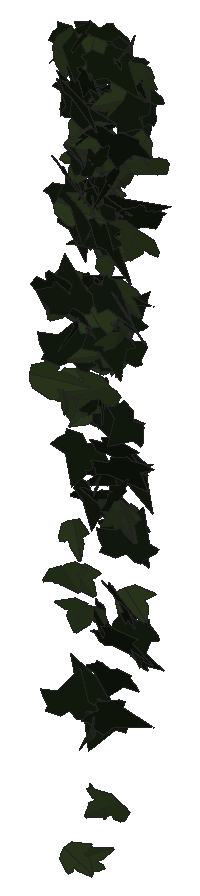
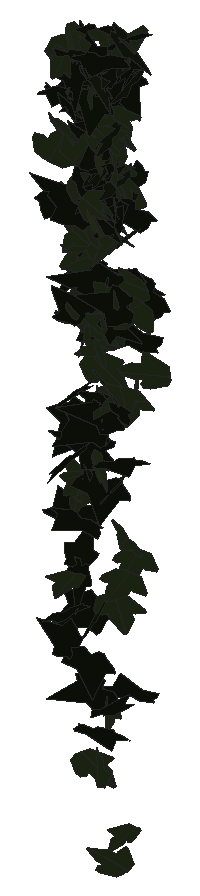
# SketchUp Ruby script. Lengths in inches.
U = 1.inch
M = Sketchup.active_model
def pt(a) = Geom::Point3d.new(a.map { |v| v * U })
def face(e, loops, mat)
  f = e.add_face(loops[0].map { |a| pt(a) })
  loops[1..].each { |l| e.add_face(l.map { |a| pt(a) }).erase! }
  f.material = f.back_material = mat if mat
  f
end
# faces: each face lists its corners as indices into pts; further lists are holes
def faces(e, pts, list, mat = nil) = list.each { |f| face(e, (f[0].is_a?(Array) ? f : [f]).map { |l| l.map { |i| pts[i] } }, mat) }
# xy, xz, yz: faces in a plane at the given z, y or x. An outline is a flat list of corners, or four numbers for a rectangle; further outlines are holes
def ring(l) = l.size == 4 ? [[l[0], l[1]], [l[2], l[1]], [l[2], l[3]], [l[0], l[3]]] : l.each_slice(2).to_a
def flat(e, list, mat, &to3) = list.each { |f| face(e, (f[0].is_a?(Array) ? f : [f]).map { |l| ring(l).map { |u, v| to3.(u, v) } }, mat) }
def xy(e, z, list, mat = nil) = flat(e, list, mat) { |x, y| [x, y, z] }
def xz(e, y, list, mat = nil) = flat(e, list, mat) { |x, z| [x, y, z] }
def yz(e, x, list, mat = nil) = flat(e, list, mat) { |y, z| [x, y, z] }
def lines(e, pts, list) = list.each { |a, b| e.add_line(pt(pts[a]), pt(pts[b])) }
# prism: a flat outline (further loops are holes) pulled along v
def prism(e, loops, v, mat = nil)
  f = face(e, loops, mat); d = Geom::Vector3d.new(v.map { |x| x * U })
  f.pushpull(f.normal.samedirection?(d) ? d.length : -d.length)
end
def box(e, o, s, mat = nil) = prism(e, [[o, [o[0] + s[0], o[1], o[2]], [o[0] + s[0], o[1] + s[1], o[2]], [o[0], o[1] + s[1], o[2]]]], [0, 0, s[2]], mat)
def at(x, y, z, deg = 0) = Geom::Transformation.translation(pt([x, y, z])) * Geom::Transformation.rotation(ORIGIN, Z_AXIS, deg.degrees)
def axes(o, x, y, z) = Geom::Transformation.new([*x, 0, *y, 0, *z, 0, *pt(o).to_a, 1])
def part(name) = M.definitions.add(name)
# library, detail: a bought-in or finely detailed component or shape, given as its bounding box
def library(name, o, s) = part(name).tap { |d| box(d.entities, o, s) }
def detail(e, o, s) = box(e.add_group.entities, o, s)
def put(e, d, t, mat = nil) = e.add_instance(d, t).tap { |i| i.material = mat if mat }
def group(e, t, mat = nil) = e.add_group.tap { |g| g.transformation = t; g.material = mat if mat }.entities
root = M.entities
M.materials.add("1026 AP 7946 SUNNY SIDE UP").color = [254, 231, 186]
M.materials.add("efeu1").color = [18, 25, 13]
M.materials.add("efeu2").color = [43, 57, 29]
c1 = part("ivyleaf_9")
p = [[1.54,2.16,1.25],[1.36,2.04,1.19],[-0.21,0.99,0.68],[-0.71,1.11,0.82],[-0.85,0.86,0.67],[-0.8,0.17,0.21],
  [-0.9,-0.01,0.1],[-0.67,-0.16,-0.02],[-0.08,-0.08,-0.05],[-0.03,-0.6,-0.4],[0.65,-0.88,-0.66],[0.83,-0.6,-0.49],
  [1.29,-0.42,-0.43],[1.8125,-0.07,-0.26],[1.21,0.44,0.15]]
faces(c1.entities,p,[[0,1,2,3,4,5,6,7,8,9,10,11,12,13,14]],"efeu1")
c2 = part("ivyleaf_10")
p = [[0,0.5,-0.03],[-0.0625,2.02,-0.43],[-0.19,2.01,-0.46],[-0.54,1.05,-0.29],[-0.52,0.625,-0.18],[-0.83,0.76,-0.28],
  [-1.16,0.64,-0.33],[-1.15,0.33,-0.24],[-0.77,-0.39,0.02],[-0.3,-0.51,0.16],[0.04,-0.48,0.23],[-0.02,2.01,-0.4375],
  [-0.06,2.01,-0.43],[0.04,-0.49,0.23],[0.67,-0.49,0.14],[1.38,0.36,-0.2],[1.375,0.51,-0.24],[0.81,0.65,-0.19],
  [0.62,0.59,-0.15],[0.6,1.09,-0.28],[0.5,1.23,-0.31]]
faces(c2.entities,p,[[0,1,2,3,4,5,6,7,8,9,10],[11,12,0,13,14,15,16,17,18,19,20]],"efeu2")
put(root,c1,axes([114.33,211.82,262.76],[-0.00033,-0.02654,-0.29608],[0.42879,0.09367,-0.00857],[0.14794,-0.27155,0.02419]),"1026 AP 7946 SUNNY SIDE UP")
put(root,c2,axes([114.36,211.6,260.97],[0.01254,0.02681,0.3018],[0.335,0.20134,-0.02379],[-0.31863,0.21274,-0.01313]),"1026 AP 7946 SUNNY SIDE UP")
put(root,c1,axes([114.53,212.3125,263.96],[0.05283,-0.25311,0.0512],[0.00752,-0.05095,-0.26333],[0.40596,0.03388,-0.00179]),"1026 AP 7946 SUNNY SIDE UP")
put(root,c1,axes([114.43,212.23,264.58],[0.0163,-0.07375,-0.26726],[0.20241,0.22903,-0.06054],[0.37195,-0.1214,0.04466]),"1026 AP 7946 SUNNY SIDE UP")
put(root,c2,axes([114.68,212.33,265.17],[0.37543,-0.0503,-0.0193],[-0.0357,-0.01866,-0.25037],[0.0763,0.23875,-0.02217]),"1026 AP 7946 SUNNY SIDE UP")
put(root,c1,axes([114.86,212.49,254.3],[-0.23794,-0.17805,0.07517],[0.05656,0.06631,0.24062],[-0.29784,0.15483,-0.01435]),"1026 AP 7946 SUNNY SIDE UP")
put(root,c2,axes([114.63,211.9375,260.46],[-0.16039,0.14591,0.17325],[0.16301,-0.13156,0.1825],[0.30873,0.14527,-0.00635]),"1026 AP 7946 SUNNY SIDE UP")
put(root,c2,axes([114.74,211.63,267.7],[-0.08324,0.20278,0.25563],[-0.10928,0.23706,-0.21446],[-0.49046,-0.08723,0.0044]),"1026 AP 7946 SUNNY SIDE UP")
put(root,c2,axes([114.67,212.23,260.8],[0.36793,0.07961,-0.01973],[-0.01745,-0.02801,-0.2537],[-0.12773,0.23313,-0.02219]),"1026 AP 7946 SUNNY SIDE UP")
put(root,c1,axes([114.54,212.54,265.16],[0.08372,-0.2346,0.12588],[0.04917,-0.11956,-0.2485],[0.41398,0.06164,0.00406]),"1026 AP 7946 SUNNY SIDE UP")
put(root,c1,axes([114.47,212.09,264.97],[0.21612,-0.20264,0.12668],[0.08618,-0.11248,-0.25238],[0.36358,0.14712,-0.01548]),"1026 AP 7946 SUNNY SIDE UP")
put(root,c2,axes([114.53,212.5625,265.2],[0.08758,-0.0713,0.2423],[0.29426,-0.14466,-0.09152],[0.25145,0.19413,0.02271]),"1026 AP 7946 SUNNY SIDE UP")
put(root,c2,axes([114.8,211.98,260.54],[-0.40626,-0.08288,0.02084],[-0.01696,-0.03377,-0.27815],[0.13324,-0.25699,0.02815]),"1026 AP 7946 SUNNY SIDE UP")
put(root,c1,axes([114.6,212.53,264.3],[-0.03694,-0.00983,0.26946],[0.05812,-0.26016,-0.00817],[0.40753,0.03621,0.02559]),"1026 AP 7946 SUNNY SIDE UP")
put(root,c1,axes([114.89,212.07,267.89],[-0.28619,0.1571,-0.11604],[0.10185,-0.09749,-0.24652],[-0.28726,-0.19108,0.02821]),"1026 AP 7946 SUNNY SIDE UP")
put(root,c1,axes([114.73,212.36,259.39],[-0.23447,-0.21161,-0.00629],[0.02595,-0.00564,-0.26616],[0.33181,-0.14909,0.01637]),"1026 AP 7946 SUNNY SIDE UP")
put(root,c1,axes([114.58,212.3,262.59],[0.12474,0.16786,-0.16247],[0.02669,0.16306,0.18742],[0.3622,-0.06983,0.04214]),"1026 AP 7946 SUNNY SIDE UP")
put(root,c2,axes([114.64,212.38,264.49],[0.21264,-0.16234,0.19252],[0.18389,-0.14697,-0.2185],[0.34429,0.17876,-0.0022]),"1026 AP 7946 SUNNY SIDE UP")
put(root,c2,axes([114.59,211.98,262.4],[-0.28318,-0.13528,-0.22766],[0.31958,0.09168,-0.22871],[0.25105,-0.2693,0.03435]),"1026 AP 7946 SUNNY SIDE UP")
put(root,c2,axes([114.7,212.1,256.93],[-0.28135,-0.14537,-0.11809],[0.17248,0.04376,-0.235],[0.23349,-0.20749,0.03131]),"1026 AP 7946 SUNNY SIDE UP")
put(root,c2,axes([114.61,212.15,257.77],[0.30253,-0.05646,0.16587],[0.22686,-0.07661,-0.20532],[0.14411,0.23911,-0.025]),"1026 AP 7946 SUNNY SIDE UP")
put(root,c1,axes([114.84,211.77,254.35],[-0.32827,0.01537,0.1306],[0.20064,0.02171,0.21404],[0.00283,0.24323,-0.02592]),"1026 AP 7946 SUNNY SIDE UP")
put(root,c2,axes([114.78,211.7,257.17],[-0.25204,-0.16994,-0.10612],[0.13137,0.06108,-0.23964],[0.28264,-0.17993,0.01676]),"1026 AP 7946 SUNNY SIDE UP")
put(root,c2,axes([114.98,212.04,256.31],[-0.37933,-0.09776,0.08145],[-0.10045,-0.05342,-0.26729],[0.17091,-0.24836,0.02369]),"1026 AP 7946 SUNNY SIDE UP")
put(root,c1,axes([114.77,212.05,267.81],[-0.09165,-0.25481,0.01381],[0.00442,-0.01587,-0.2693],[0.40131,-0.05802,0.00612]),"1026 AP 7946 SUNNY SIDE UP")
put(root,c2,axes([114.8125,212.31,263.83],[-0.01325,0.17298,0.19125],[-0.0111,0.18453,-0.17733],[-0.3977,-0.01092,-0.00142]),"1026 AP 7946 SUNNY SIDE UP")
put(root,c2,axes([114.97,212.18,265.3],[-0.42627,0.09776,-0.06355],[-0.08046,0.0411,0.29635],[0.1635,0.27509,-0.01985]),"1026 AP 7946 SUNNY SIDE UP")
put(root,c1,axes([115.01,211.63,262.65],[-0.44689,0.03987,0.0216],[0.03714,0.01954,0.29485],[0.06012,0.28429,-0.02159]),"1026 AP 7946 SUNNY SIDE UP")
put(root,c2,axes([115.05,212.33,265.92],[-0.24515,-0.10156,0.16635],[-0.14571,-0.14278,-0.18486],[0.26306,-0.17373,0.05263]),"1026 AP 7946 SUNNY SIDE UP")
put(root,c2,axes([115.02,212.12,266.26],[-0.29988,-0.12456,0.12883],[-0.09785,-0.12589,-0.22639],[0.26055,-0.19063,0.06326]),"1026 AP 7946 SUNNY SIDE UP")
put(root,c1,axes([115.02,212.05,266.45],[0.10534,0.08239,0.2645],[-0.36305,-0.1182,0.10063],[0.21764,-0.23705,0.03985]),"1026 AP 7946 SUNNY SIDE UP")
put(root,c2,axes([114.58,211.92,262.8125],[-0.04554,-0.04058,-0.28364],[0.41006,-0.09998,-0.01367],[-0.15179,-0.25792,0.04816]),"1026 AP 7946 SUNNY SIDE UP")
put(root,c1,axes([114.76,212.37,265.35],[0.04224,-0.16714,-0.2027],[0.01587,0.19741,-0.17101],[0.4045,0.00971,0.02788]),"1026 AP 7946 SUNNY SIDE UP")
put(root,c2,axes([114.76,212.2,251.09],[-0.15756,-0.10948,0.19911],[0.17686,0.15862,0.15308],[-0.30217,0.14992,-0.01423]),"1026 AP 7946 SUNNY SIDE UP")
put(root,c1,axes([115,212.14,262.17],[-0.13648,0.11021,-0.22666],[0.13675,-0.2052,-0.14204],[-0.3629,-0.11877,0.03171]),"1026 AP 7946 SUNNY SIDE UP")
put(root,c1,axes([114.91,211.74,261.48],[-0.38073,0.00603,0.1913],[0.29141,-0.0128,0.24935],[0.01977,0.30485,0.00848]),"1026 AP 7946 SUNNY SIDE UP")
put(root,c2,axes([115.02,212.24,260.35],[0.16107,0.12713,-0.20432],[-0.17254,-0.16652,-0.16871],[-0.32888,0.14963,-0.01156]),"1026 AP 7946 SUNNY SIDE UP")
put(root,c2,axes([114.92,212.52,265.6],[0.06572,-0.21079,0.17182],[0.08258,-0.16036,-0.2217],[0.4157,0.06518,0.01688]),"1026 AP 7946 SUNNY SIDE UP")
put(root,c1,axes([114.97,212.62,253.97],[-0.31181,-0.13764,-0.05804],[0.08965,0.01497,-0.24776],[0.21548,-0.2054,0.01909]),"1026 AP 7946 SUNNY SIDE UP")
put(root,c2,axes([115.01,212.31,262.73],[-0.35127,0.10195,0.01562],[-0.03524,-0.01411,-0.25203],[-0.15806,-0.22343,0.02147]),"1026 AP 7946 SUNNY SIDE UP")
put(root,c1,axes([114.84,212.62,267.7],[-0.15084,-0.20268,-0.14255],[0.12253,0.11442,-0.22956],[0.36483,-0.12223,0.01816]),"1026 AP 7946 SUNNY SIDE UP")
put(root,c1,axes([115.11,211.89,266.95],[0.16197,0.14313,-0.21774],[-0.16676,-0.18428,-0.18219],[-0.36626,0.1472,-0.01334]),"1026 AP 7946 SUNNY SIDE UP")
put(root,c1,axes([114.74,211.9375,266.87],[0.18109,-0.24615,0.08068],[0.04699,-0.07401,-0.28037],[0.40411,0.11891,-0.00355]),"1026 AP 7946 SUNNY SIDE UP")
put(root,c1,axes([114.77,212.44,265.99],[0.20692,-0.21471,0.044],[0.02556,-0.04153,-0.25956],[0.34366,0.13237,-0.00719]),"1026 AP 7946 SUNNY SIDE UP")
put(root,c1,axes([114.86,212.12,264.56],[-0.01671,-0.28823,0.10739],[-0.0139,-0.10561,-0.29771],[0.48262,-0.01302,-0.00485]),"1026 AP 7946 SUNNY SIDE UP")
put(root,c1,axes([114.83,212.5625,265.42],[0.25776,-0.18658,-0.05448],[-0.06224,0.03418,-0.25556],[0.29806,0.16849,-0.00625]),"1026 AP 7946 SUNNY SIDE UP")
put(root,c2,axes([114.75,211.8,264.5],[0.07882,0.08024,0.25324],[0.2894,0.16415,-0.09308],[-0.28463,0.18913,-0.02451]),"1026 AP 7946 SUNNY SIDE UP")
put(root,c2,axes([115.0625,212.7,264.71],[-0.04653,-0.17889,0.16621],[-0.00601,-0.1632,-0.18693],[0.37981,-0.0245,0.0174]),"1026 AP 7946 SUNNY SIDE UP")
put(root,c1,axes([115.04,211.72,267.4],[0.32511,-0.00899,-0.16815],[-0.25595,-0.03466,-0.21072],[-0.02278,0.2611,-0.0322]),"1026 AP 7946 SUNNY SIDE UP")
put(root,c2,axes([115.04,212.62,264.47],[0.10511,-0.2419,0.06588],[0.02007,-0.06423,-0.25887],[0.39348,0.06789,-0.00439]),"1026 AP 7946 SUNNY SIDE UP")
put(root,c2,axes([115.2,212.02,265.97],[0.27421,-0.06713,-0.17344],[-0.26623,0.02155,-0.18984],[0.10012,0.24117,-0.02978]),"1026 AP 7946 SUNNY SIDE UP")
put(root,c1,axes([115.27,212.01,260.68],[-0.25317,0.0472,-0.20083],[-0.27572,0.08894,0.17167],[0.15396,0.2369,-0.0228]),"1026 AP 7946 SUNNY SIDE UP")
put(root,c2,axes([114.94,211.68,251.5],[0.06808,0.1999,0.15334],[0.06439,0.14215,-0.20972],[-0.38549,0.05905,-0.00795]),"1026 AP 7946 SUNNY SIDE UP")
put(root,c1,axes([115.25,212.3125,267.04],[-0.07873,0.21785,0.15019],[-0.08554,0.13528,-0.22865],[-0.4021,-0.07143,0.01923]),"1026 AP 7946 SUNNY SIDE UP")
put(root,c1,axes([115.08,212.39,264.43],[-0.34316,-0.00683,-0.13327],[0.20333,-0.02535,-0.22357],[-0.01114,-0.25241,0.02457]),"1026 AP 7946 SUNNY SIDE UP")
put(root,c1,axes([114.73,212.42,264.47],[0.16533,-0.08289,0.2334],[0.26394,-0.15309,-0.13856],[0.27342,0.1979,-0.00737]),"1026 AP 7946 SUNNY SIDE UP")
put(root,c1,axes([114.96,212.5625,264.34],[-0.25664,-0.06035,-0.19575],[0.296,0.03285,-0.17746],[0.10164,-0.24806,0.02256]),"1026 AP 7946 SUNNY SIDE UP")
put(root,c1,axes([115.1875,212.21,260.18],[-0.00212,-0.01033,0.27381],[0.01914,0.26557,0.01225],[-0.4179,0.01221,-0.00083]),"1026 AP 7946 SUNNY SIDE UP")
put(root,c1,axes([114.9,212.23,267.1],[0.02279,-0.23983,0.14183],[0.07843,-0.1347,-0.24551],[0.42879,0.03738,0.03737]),"1026 AP 7946 SUNNY SIDE UP")
put(root,c1,axes([115.01,212.01,265.875],[0.02431,0.20522,-0.14568],[-0.02947,0.1434,0.21138],[0.39181,-0.00194,0.02494]),"1026 AP 7946 SUNNY SIDE UP")
put(root,c1,axes([115.12,212.13,264.85],[-0.03383,0.01205,-0.27123],[-0.12928,0.25074,0.02021],[0.39385,0.08334,-0.01666]),"1026 AP 7946 SUNNY SIDE UP")
put(root,c1,axes([115.02,212.17,258.57],[0.00573,-0.21449,0.14752],[0.00012,-0.14443,-0.22184],[0.40659,0.00306,-0.00201]),"1026 AP 7946 SUNNY SIDE UP")
put(root,c2,axes([115.08,212.07,267.76],[0.42022,0.00669,0.01111],[0.01787,-0.02704,-0.27412],[-0.00875,0.26609,-0.02656]),"1026 AP 7946 SUNNY SIDE UP")
put(root,c1,axes([114.97,212.29,266.96],[0.02013,-0.11405,0.27966],[0.04872,-0.27034,-0.11981],[0.46137,0.03352,0.00045]),"1026 AP 7946 SUNNY SIDE UP")
put(root,c1,axes([115.18,212.08,258.7],[0.26933,0.16506,-0.09544],[-0.09338,-0.0731,-0.24524],[-0.28336,0.18098,-0.0099]),"1026 AP 7946 SUNNY SIDE UP")
put(root,c2,axes([115.45,211.96,260.98],[-0.28177,-0.04094,0.22446],[-0.32075,-0.08003,-0.18859],[0.13744,-0.2707,0.02005]),"1026 AP 7946 SUNNY SIDE UP")
put(root,c1,axes([114.99,212.25,260.46],[-0.15882,-0.09946,-0.22489],[0.27963,0.12702,-0.14402],[0.25196,-0.20366,0.01808]),"1026 AP 7946 SUNNY SIDE UP")
put(root,c1,axes([115.23,212.33,266.67],[0.08555,0.24449,0.04203],[0.0228,0.03713,-0.25774],[-0.38873,0.05599,-0.00587]),"1026 AP 7946 SUNNY SIDE UP")
put(root,c1,axes([114.87,212.21,260.2],[0.2289,0.03134,0.21507],[0.33136,-0.01063,-0.14993],[-0.01436,0.25414,-0.03128]),"1026 AP 7946 SUNNY SIDE UP")
put(root,c2,axes([115.22,212.31,266.68],[0.0081,-0.22943,0.10885],[0.02653,-0.10643,-0.23665],[0.39715,0.01179,0.01359]),"1026 AP 7946 SUNNY SIDE UP")
put(root,c2,axes([115.27,211.81,254.05],[-0.00155,-0.18355,-0.18483],[-0.01435,0.17829,-0.18791],[0.4022,0.00565,-0.00742]),"1026 AP 7946 SUNNY SIDE UP")
put(root,c1,axes([115.11,212.28,265.08],[0.32226,-0.18291,-0.06628],[0.09619,-0.02626,0.28204],[-0.28874,-0.21289,0.01998]),"1026 AP 7946 SUNNY SIDE UP")
put(root,c1,axes([115.17,212.17,256.26],[0.22429,-0.14788,-0.15397],[-0.18841,0.09,-0.21021],[0.27052,0.18529,-0.01875]),"1026 AP 7946 SUNNY SIDE UP")
put(root,c2,axes([115.26,212.22,259.14],[0.13125,-0.24883,0.03075],[0.00478,-0.03194,-0.27047],[0.39431,0.08322,-0.00696]),"1026 AP 7946 SUNNY SIDE UP")
put(root,c2,axes([115.02,212.47,264.52],[-0.20653,-0.02957,-0.20903],[0.31659,-0.06318,-0.12526],[-0.0596,-0.23315,0.05896]),"1026 AP 7946 SUNNY SIDE UP")
put(root,c2,axes([115.21,212.26,263.93],[0.26447,0.17563,-0.03517],[-0.01991,-0.03641,-0.25019],[-0.28092,0.16792,-0.01537]),"1026 AP 7946 SUNNY SIDE UP")
put(root,c1,axes([115.07,211.97,266.64],[0.04419,-0.03717,-0.2968],[0.09254,0.28396,-0.03019],[0.44696,-0.05512,0.03559]),"1026 AP 7946 SUNNY SIDE UP")
put(root,c1,axes([114.93,212.15,262.78],[0.16576,0.08648,-0.27029],[0.28541,0.19071,0.14075],[0.32843,-0.20938,0.0141]),"1026 AP 7946 SUNNY SIDE UP")
put(root,c1,axes([115.56,212.07,264.05],[-0.34156,0.10529,0.0541],[-0.09154,-0.00179,-0.2472],[-0.1603,-0.22333,0.02589]),"1026 AP 7946 SUNNY SIDE UP")
put(root,c2,axes([115.55,212.125,261.83],[0.14327,-0.04614,-0.23695],[-0.33665,0.0838,-0.10432],[0.14977,0.23251,-0.00783]),"1026 AP 7946 SUNNY SIDE UP")
put(root,c2,axes([115.375,212.64,264.96],[-0.06121,-0.19596,0.14744],[-0.02907,-0.14326,-0.20649],[0.38148,-0.04236,0.00792]),"1026 AP 7946 SUNNY SIDE UP")
put(root,c2,axes([115.49,211.97,261.7],[-0.04619,-0.04949,0.26592],[-0.17938,-0.23191,-0.06047],[0.3728,-0.11772,0.00385]),"1026 AP 7946 SUNNY SIDE UP")
put(root,c2,axes([115.22,212.03,261.42],[0.28314,0.1858,-0.16773],[0.1545,0.1324,0.26666],[0.3576,-0.20432,0.01759]),"1026 AP 7946 SUNNY SIDE UP")
put(root,c1,axes([115.03,212.47,265.53],[0.32902,-0.03706,-0.16486],[0.25312,-0.00358,0.21797],[-0.04976,-0.26327,0.01867]),"1026 AP 7946 SUNNY SIDE UP")
put(root,c2,axes([115.45,212.12,261.66],[0.2617,-0.15377,-0.15136],[-0.13687,0.11977,-0.23139],[0.30409,0.18624,0.02612]),"1026 AP 7946 SUNNY SIDE UP")
put(root,c2,axes([115.5,212.47,265.44],[-0.19124,-0.17251,-0.22249],[-0.22357,-0.16206,0.21587],[-0.37132,0.18642,-0.01539]),"1026 AP 7946 SUNNY SIDE UP")
put(root,c1,axes([115.41,212.21,255.125],[0.27747,0.08269,-0.15483],[-0.19855,-0.08432,-0.20039],[-0.18353,0.21624,-0.0173]),"1026 AP 7946 SUNNY SIDE UP")
put(root,c1,axes([115.52,211.65,265.64],[-0.00992,0.15814,0.22183],[-0.05873,0.21184,-0.16085],[-0.41481,-0.03377,0.01747]),"1026 AP 7946 SUNNY SIDE UP")
put(root,c1,axes([115.41,212.45,265.1875],[-0.17006,0.1098,-0.26555],[0.23735,-0.21074,-0.15857],[-0.37223,-0.18454,0.02021]),"1026 AP 7946 SUNNY SIDE UP")
put(root,c2,axes([115.12,212.38,261.97],[-0.12764,0.03456,0.24926],[0.38223,-0.01303,0.08593],[0.03687,0.25469,-0.0279]),"1026 AP 7946 SUNNY SIDE UP")
put(root,c2,axes([115.27,211.91,262.4],[0.20464,0.21282,0.09279],[0.09199,0.06823,-0.25622],[-0.35078,0.14205,-0.01306]),"1026 AP 7946 SUNNY SIDE UP")
put(root,c1,axes([115.57,212.24,267.09],[-0.15557,0.16313,-0.16999],[0.05083,-0.16893,-0.19193],[-0.36234,-0.09373,0.04606]),"1026 AP 7946 SUNNY SIDE UP")
put(root,c2,axes([115.46,212.6,263.93],[0.06522,0.18216,-0.15996],[-0.1103,-0.1425,-0.1911],[-0.36095,0.07646,0.02949]),"1026 AP 7946 SUNNY SIDE UP")
put(root,c1,axes([115.27,212.32,267.26],[-0.10385,-0.02201,0.26335],[0.15705,-0.24548,0.00337],[0.37183,0.09753,0.07213]),"1026 AP 7946 SUNNY SIDE UP")
put(root,c1,axes([115.42,212.2,261.71],[0.20921,-0.24674,-0.03846],[0.05213,-0.02286,0.28804],[-0.38858,-0.13591,0.01794]),"1026 AP 7946 SUNNY SIDE UP")
put(root,c2,axes([115.4,211.94,252.52],[-0.25823,0.14004,0.1238],[0.16552,-0.05974,0.22104],[0.23732,0.19404,-0.01946]),"1026 AP 7946 SUNNY SIDE UP")
put(root,c1,axes([115.6,212.52,267.48],[-0.38935,-0.10149,0.01712],[-0.00946,-0.03044,-0.27457],[0.16158,-0.24633,0.02517]),"1026 AP 7946 SUNNY SIDE UP")
put(root,c1,axes([115.6,212.48,267.22],[0.24564,0.00293,-0.22428],[-0.34229,0.00846,-0.16074],[0.00812,0.26784,0.0091]),"1026 AP 7946 SUNNY SIDE UP")
put(root,c1,axes([115.51,211.95,262.97],[0.35153,-0.03961,-0.16663],[-0.25531,0.00656,-0.23314],[0.05657,0.27573,-0.01674]),"1026 AP 7946 SUNNY SIDE UP")
put(root,c2,axes([115.4,212.04,263.63],[0.04957,-0.08096,-0.31813],[0.2279,0.27961,-0.05873],[0.44647,-0.13374,0.0653]),"1026 AP 7946 SUNNY SIDE UP")
put(root,c2,axes([115.42,212.45,266.54],[0.04515,-0.25097,-0.09404],[0.09816,-0.08153,0.25467],[-0.4075,-0.04744,0.05093]),"1026 AP 7946 SUNNY SIDE UP")
put(root,c2,axes([115.79,211.8125,252.73],[-0.26988,-0.05917,0.19223],[-0.25953,-0.09051,-0.18616],[0.16643,-0.23709,0.02142]),"1026 AP 7946 SUNNY SIDE UP")
put(root,c2,axes([115.61,212.39,262.41],[-0.03525,-0.16609,0.20332],[-0.01052,-0.19861,-0.17331],[0.4066,-0.01954,0.01314]),"1026 AP 7946 SUNNY SIDE UP")
put(root,c1,axes([115.8,212.03,261.67],[-0.46631,-0.04905,0.01677],[0.01945,0.02635,0.30883],[-0.07904,0.29585,-0.02294]),"1026 AP 7946 SUNNY SIDE UP")
put(root,c1,axes([115.37,211.99,254.39],[0.06645,0.03095,-0.26148],[0.10017,0.24805,0.04351],[0.38966,-0.06904,0.03341]),"1026 AP 7946 SUNNY SIDE UP")
put(root,c1,axes([115.67,212.11,261.39],[-0.02933,-0.12034,0.23658],[0.06432,0.22668,0.12675],[-0.40353,0.04488,0.00301]),"1026 AP 7946 SUNNY SIDE UP")
put(root,c1,axes([115.37,211.91,259.21],[0.16771,0.19803,-0.14556],[0.0556,0.14125,0.23043],[0.37949,-0.10821,0.03057]),"1026 AP 7946 SUNNY SIDE UP")
put(root,c1,axes([115.47,212.36,262.11],[-0.15945,-0.03808,0.24361],[0.36175,0.05678,0.11129],[-0.10596,0.25116,0.01335]),"1026 AP 7946 SUNNY SIDE UP")
put(root,c1,axes([115.41,211.99,264.16],[0.227,-0.27253,-0.00539],[-0.02188,-0.00321,-0.31742],[0.42801,0.14437,-0.01337]),"1026 AP 7946 SUNNY SIDE UP")
put(root,c1,axes([115.44,212.05,259.8],[0.40024,0.04172,0.03509],[0.05884,-0.02023,-0.26451],[-0.06058,0.25598,-0.02508]),"1026 AP 7946 SUNNY SIDE UP")
put(root,c2,axes([115.72,212.36,267.8],[0.04802,-0.26247,-0.05086],[-0.01846,0.04683,-0.27188],[0.41912,0.03213,-0.00614]),"1026 AP 7946 SUNNY SIDE UP")
put(root,c1,axes([115.33,212.46,264.37],[0.33986,0.12705,-0.13737],[0.15562,0.09458,0.25726],[0.24522,-0.2361,0.02713]),"1026 AP 7946 SUNNY SIDE UP")
put(root,c2,axes([115.55,212.125,258.52],[-0.39613,0.06084,-0.13972],[0.19739,-0.05711,-0.26627],[-0.12609,-0.28053,0.02212]),"1026 AP 7946 SUNNY SIDE UP")
put(root,c1,axes([115.73,212.07,256.74],[0.25903,-0.04697,-0.20444],[-0.30584,0.03933,-0.17593],[0.095,0.25469,-0.00896]),"1026 AP 7946 SUNNY SIDE UP")
put(root,c1,axes([115.48,212.43,258.01],[-0.1069,-0.12029,-0.21136],[0.26563,0.1248,-0.13277],[0.26191,-0.17567,0.04838]),"1026 AP 7946 SUNNY SIDE UP")
put(root,c1,axes([115.52,211.93,267.73],[0.03586,-0.18858,-0.19756],[0.0436,0.19202,-0.19108],[0.41945,-0.00384,0.03676]),"1026 AP 7946 SUNNY SIDE UP")
put(root,c2,axes([115.73,212.12,266.84],[-0.02356,0.04059,0.30487],[0.0138,-0.29589,0.04057],[0.46913,0.01074,0.01412]),"1026 AP 7946 SUNNY SIDE UP")
put(root,c1,axes([115.47,212.03,255.98],[0.39551,0.02226,0.06388],[0.10007,-0.02071,-0.25893],[-0.02607,0.2582,-0.02474]),"1026 AP 7946 SUNNY SIDE UP")
put(root,c2,axes([115.73,212.12,258.47],[-0.14735,-0.23123,-0.08535],[0.06385,0.07145,-0.2564],[0.38021,-0.10161,0.00998]),"1026 AP 7946 SUNNY SIDE UP")
put(root,c2,axes([115.625,211.8125,261.81],[0.09141,0.05326,-0.26427],[0.16845,0.2353,0.07663],[0.37646,-0.11822,0.02988]),"1026 AP 7946 SUNNY SIDE UP")
put(root,c1,axes([115.87,211.74,258.95],[-0.02068,0.18598,0.19576],[-0.02116,0.18849,-0.19097],[-0.41637,-0.01881,-0.00002]),"1026 AP 7946 SUNNY SIDE UP")
put(root,c1,axes([115.62,211.89,262.12],[-0.0958,-0.21251,-0.10876],[0.06027,0.09749,-0.22699],[0.36736,-0.07141,0.00887]),"1026 AP 7946 SUNNY SIDE UP")
put(root,c1,axes([115.59,212.52,259.27],[0.13087,-0.26147,-0.10331],[-0.06377,0.09069,-0.28194],[0.43485,0.09199,-0.01026]),"1026 AP 7946 SUNNY SIDE UP")
put(root,c2,axes([115.86,212.26,267.48],[-0.36187,-0.12771,0.05526],[-0.05264,-0.05109,-0.26992],[0.21181,-0.23089,0.02733]),"1026 AP 7946 SUNNY SIDE UP")
put(root,c2,axes([115.81,211.88,262.1875],[-0.09758,-0.23601,0.02266],[0.00106,-0.0243,-0.25145],[0.37292,-0.06169,0.00664]),"1026 AP 7946 SUNNY SIDE UP")
put(root,c1,axes([115.65,212.62,266.78],[-0.09357,-0.23139,-0.10246],[0.07719,0.08821,-0.24441],[0.3876,-0.07343,0.02394]),"1026 AP 7946 SUNNY SIDE UP")
put(root,c1,axes([115.83,211.79,266.28],[0.36403,0.11664,-0.16444],[-0.20635,-0.09452,-0.26669],[-0.23362,0.26524,-0.02067]),"1026 AP 7946 SUNNY SIDE UP")
put(root,c1,axes([115.67,211.71,263.2],[0.14765,-0.19221,-0.17033],[-0.07665,0.15815,-0.21846],[0.39008,0.10383,0.02155]),"1026 AP 7946 SUNNY SIDE UP")
put(root,c2,axes([115.95,212.59,265.34],[-0.39527,-0.09148,-0.10178],[-0.15334,-0.01899,0.27507],[-0.14512,0.26924,-0.01342]),"1026 AP 7946 SUNNY SIDE UP")
put(root,c1,axes([115.96,212.49,264.47],[-0.02214,0.12577,-0.22513],[-0.02413,-0.21961,-0.13005],[-0.39671,0.00634,0.02047]),"1026 AP 7946 SUNNY SIDE UP")
put(root,c1,axes([115.83,212.29,260.3],[-0.1339,-0.17723,0.18297],[-0.08949,-0.17012,-0.20284],[0.3854,-0.10108,0.01647]),"1026 AP 7946 SUNNY SIDE UP")
put(root,c1,axes([115.86,212.58,266.57],[-0.34271,0.01054,-0.13247],[0.20016,-0.0243,-0.22437],[-0.03365,-0.25192,0.0146]),"1026 AP 7946 SUNNY SIDE UP")
put(root,c2,axes([115.71,212.37,256.7],[0.17288,0.20014,0.09759],[0.08199,0.07809,-0.23466],[-0.33759,0.12145,-0.00701]),"1026 AP 7946 SUNNY SIDE UP")
put(root,c1,axes([115.74,212.53,256.0625],[-0.06979,-0.24551,-0.01315],[0.01546,0.00977,-0.25683],[0.38614,-0.04476,0.00791]),"1026 AP 7946 SUNNY SIDE UP")
put(root,c2,axes([115.89,212.49,265.91],[0.34316,-0.16128,-0.05444],[-0.08265,0.01605,-0.27885],[0.25327,0.22376,-0.01723]),"1026 AP 7946 SUNNY SIDE UP")
put(root,c2,axes([115.69,212.02,263.08],[-0.30836,0.04632,-0.16294],[0.23199,-0.06111,-0.20691],[-0.11636,-0.24459,0.01927]),"1026 AP 7946 SUNNY SIDE UP")
put(root,c1,axes([115.57,212.59,255.47],[0.12493,-0.09023,0.22504],[0.1992,-0.17893,-0.12437],[0.31462,0.14912,-0.01062]),"1026 AP 7946 SUNNY SIDE UP")
put(root,c1,axes([116.1875,211.97,266.73],[-0.26255,0.11938,0.15768],[-0.25308,0.02619,-0.20267],[-0.16911,-0.22453,0.05849]),"1026 AP 7946 SUNNY SIDE UP")
put(root,c2,axes([115.83,212.0625,258.65],[-0.25497,0.19397,-0.07331],[0.05225,-0.06621,-0.2603],[-0.32126,-0.16472,0.01585]),"1026 AP 7946 SUNNY SIDE UP")
put(root,c2,axes([115.87,212.46,267.29],[-0.32184,0.14326,-0.05565],[0.04894,-0.05075,-0.25657],[-0.23618,-0.20573,0.02268]),"1026 AP 7946 SUNNY SIDE UP")
put(root,c1,axes([115.875,212.09,257.77],[-0.31419,-0.03015,0.19677],[0.29637,0.0321,0.20835],[-0.06912,0.27467,-0.00111]),"1026 AP 7946 SUNNY SIDE UP")
put(root,c2,axes([116.07,212.13,264.22],[-0.44889,0.02813,0.09341],[-0.14573,-0.02259,-0.29402],[-0.03126,-0.29863,0.02926]),"1026 AP 7946 SUNNY SIDE UP")
put(root,c1,axes([115.79,211.93,262.875],[0.35876,-0.1287,-0.09992],[-0.15074,0.02517,-0.26861],[0.20282,0.24635,-0.0229]),"1026 AP 7946 SUNNY SIDE UP")
put(root,c1,axes([115.88,211.92,256.8125],[0.27632,-0.17674,0.02008],[-0.00361,0.02656,0.25632],[-0.27975,-0.17492,0.01653]),"1026 AP 7946 SUNNY SIDE UP")
put(root,c1,axes([115.79,211.78,259.64],[0.39004,0.16297,0.02031],[0.04509,-0.00954,-0.30484],[-0.25398,0.24858,-0.02293]),"1026 AP 7946 SUNNY SIDE UP")
